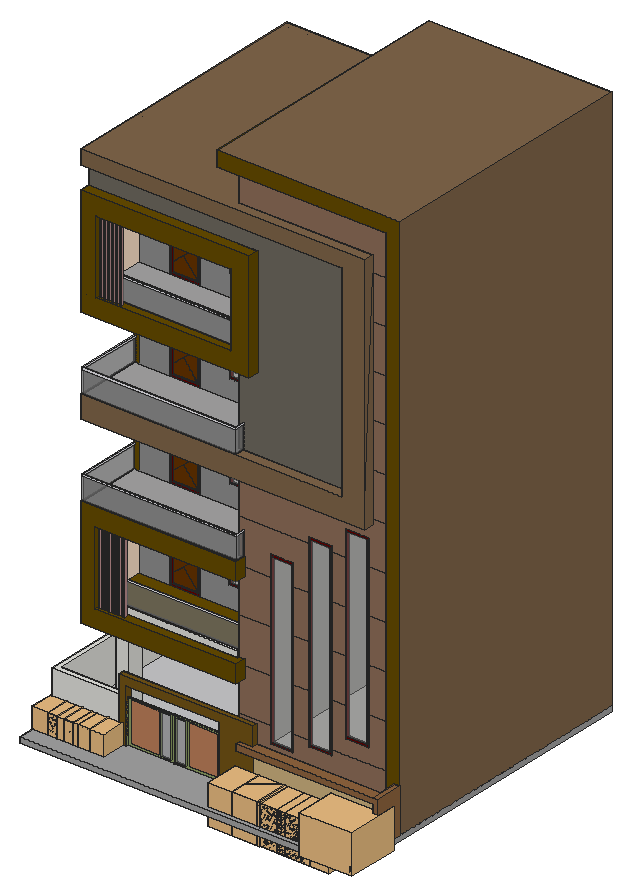
# SketchUp Ruby script. Lengths in inches.
U = 1.inch
M = Sketchup.active_model
def pt(a) = Geom::Point3d.new(a.map { |v| v * U })
def face(e, loops, mat)
  f = e.add_face(loops[0].map { |a| pt(a) })
  loops[1..].each { |l| e.add_face(l.map { |a| pt(a) }).erase! }
  f.material = f.back_material = mat if mat
  f
end
# faces: each face lists its corners as indices into pts; further lists are holes
def faces(e, pts, list, mat = nil) = list.each { |f| face(e, (f[0].is_a?(Array) ? f : [f]).map { |l| l.map { |i| pts[i] } }, mat) }
# xy, xz, yz: faces in a plane at the given z, y or x. An outline is a flat list of corners, or four numbers for a rectangle; further outlines are holes
def ring(l) = l.size == 4 ? [[l[0], l[1]], [l[2], l[1]], [l[2], l[3]], [l[0], l[3]]] : l.each_slice(2).to_a
def flat(e, list, mat, &to3) = list.each { |f| face(e, (f[0].is_a?(Array) ? f : [f]).map { |l| ring(l).map { |u, v| to3.(u, v) } }, mat) }
def xy(e, z, list, mat = nil) = flat(e, list, mat) { |x, y| [x, y, z] }
def xz(e, y, list, mat = nil) = flat(e, list, mat) { |x, z| [x, y, z] }
def yz(e, x, list, mat = nil) = flat(e, list, mat) { |y, z| [x, y, z] }
def lines(e, pts, list) = list.each { |a, b| e.add_line(pt(pts[a]), pt(pts[b])) }
# prism: a flat outline (further loops are holes) pulled along v
def prism(e, loops, v, mat = nil)
  f = face(e, loops, mat); d = Geom::Vector3d.new(v.map { |x| x * U })
  f.pushpull(f.normal.samedirection?(d) ? d.length : -d.length)
end
def box(e, o, s, mat = nil) = prism(e, [[o, [o[0] + s[0], o[1], o[2]], [o[0] + s[0], o[1] + s[1], o[2]], [o[0], o[1] + s[1], o[2]]]], [0, 0, s[2]], mat)
def at(x, y, z, deg = 0) = Geom::Transformation.translation(pt([x, y, z])) * Geom::Transformation.rotation(ORIGIN, Z_AXIS, deg.degrees)
def axes(o, x, y, z) = Geom::Transformation.new([*x, 0, *y, 0, *z, 0, *pt(o).to_a, 1])
def part(name) = M.definitions.add(name)
# library, detail: a bought-in or finely detailed component or shape, given as its bounding box
def library(name, o, s) = part(name).tap { |d| box(d.entities, o, s) }
def detail(e, o, s) = box(e.add_group.entities, o, s)
def put(e, d, t, mat = nil) = e.add_instance(d, t).tap { |i| i.material = mat if mat }
def group(e, t, mat = nil) = e.add_group.tap { |g| g.transformation = t; g.material = mat if mat }.entities
root = M.entities
M.materials.add("[0040_Peru]").color = [143, 110, 89]
M.materials.add("[0040_Peru]1").color = [143, 101, 63]
M.materials.add("[0040_Peru]2").color = [205, 133, 63]
M.materials.add("[0058_Olive]").color = [128, 102, 74]
M.materials.add("[0058_Olive]1").color = [143, 161, 101]
M.materials.add("[0058_Olive]2").color = [114, 83, 22]
M.materials.add("[0119_RosyBrown]").color = [188, 143, 143]
M.materials.add("[Blacktop Old 02]").color = [143, 145, 145]
M.materials.add("[Cladding Weathered]1").color = [111, 105, 96]
M.materials.add("[Color A08]").color = [102, 0, 0]
M.materials.add("[Color B08]").color = [102, 25, 0]
M.materials.add("[Color C01]").color = [255, 229, 204]
M.materials.add("[Color C08]").color = [102, 51, 0]
M.materials.add("[Color D08]").color = [102, 76, 0]
M.materials.add("[Color M04]").color = [142, 142, 142]
M.materials.add("[Grass Dark Green]").color = [106, 157, 55]
M.materials.add("[Metal Silver]").color = [234, 233, 238]
M.materials.add("[Pavers Flagstone Gray]").color = [162, 162, 162]
M.materials.add("[Polished Concrete New]").color = [200, 200, 203]
M.materials.add("[Stone Sandstone Ashlar Light]").color = [206, 178, 128]
M.materials.add("[Stone Vein Gray]").color = [166, 165, 165]
M.materials.add("[Translucent Glass Gray]").color = [128, 128, 128]
M.materials["[Translucent Glass Gray]"].alpha = 0.5
M.materials.add("[Wood Veneer 02]").color = [190, 128, 91]
c1 = library("Flowering shrub",[-7.36,-7.49,-12.9],[86.01,85.74,63.18])
c2 = library("plant\#1",[-28.7,-9.94,-2.13],[41.67,42.29,34.27])
c3 = part("Group\#2")
xy(c3.entities,0,[[0,0,52.4375,3.1875]],"[Color A08]")
xy(c3.entities,2.41,[[2.41,0,24.62,3.1875],[26.04,0,50.02,3.1875]],"[Color A08]")
xy(c3.entities,67.21,[[2.41,0,24.62,3.1875],[26.04,0,50.02,3.1875]],"[Color A08]")
xy(c3.entities,69.625,[[0,0,52.4375,3.1875]],"[Color A08]")
xz(c3.entities,0,[[[0,0,52.4375,69.625],[26.04,2.41,50.02,67.21],[2.41,2.41,24.62,67.21]]],"[Color A08]")
xz(c3.entities,0,[[2.41,2.41,24.62,67.21],[26.04,2.41,50.02,67.21]],"[Translucent Glass Gray]")
xz(c3.entities,3.1875,[[[0,0,52.4375,69.625],[26.04,2.41,50.02,67.21],[2.41,2.41,24.62,67.21]]],"[Color A08]")
yz(c3.entities,0,[[0,0,3.1875,69.625]],"[Color A08]")
yz(c3.entities,2.41,[[0,2.41,3.1875,67.21]],"[Color A08]")
yz(c3.entities,24.62,[[0,2.41,3.1875,67.21]],"[Color A08]")
yz(c3.entities,26.04,[[0,2.41,3.1875,67.21]],"[Color A08]")
yz(c3.entities,50.02,[[0,2.41,3.1875,67.21]],"[Color A08]")
yz(c3.entities,52.4375,[[0,0,3.1875,69.625]],"[Color A08]")
c4 = part("Group\#1")
xy(c4.entities,0,[[0,0,27.5625,2.875]],"[Color A08]")
xy(c4.entities,2.09,[[2.09,0,25.47,2.875]],"[Color A08]")
xy(c4.entities,198.72,[[2.09,0,25.47,2.875]],"[Color A08]")
xy(c4.entities,200.8125,[[0,0,27.5625,2.875]],"[Color A08]")
xz(c4.entities,0,[[[0,0,27.5625,200.8125],[2.09,2.09,25.47,198.72]]],"[Color A08]")
xz(c4.entities,0,[[2.09,2.09,25.47,198.72]],"[Translucent Glass Gray]")
xz(c4.entities,2.875,[[[0,0,27.5625,200.8125],[2.09,2.09,25.47,198.72]]],"[Color A08]")
yz(c4.entities,0,[[0,0,2.875,200.8125]],"[Color A08]")
yz(c4.entities,2.09,[[0,2.09,2.875,198.72]],"[Color A08]")
yz(c4.entities,25.47,[[0,2.09,2.875,198.72]],"[Color A08]")
yz(c4.entities,27.5625,[[0,0,2.875,200.8125]],"[Color A08]")
c5 = part("Group\#3")
xy(c5.entities,0,[[0,0,48,2.4375]],"[Color A08]")
xy(c5.entities,2.92,[[2.92,0,45.08,2.4375]],"[Color A08]")
xy(c5.entities,81.08,[[2.92,0,37.65,2.4375],[37.65,0,40.5,2.4375],[40.5,0,45.08,2.4375]],"[Color B08]")
xy(c5.entities,84,[[0,0,48,2.4375]],"[Color A08]")
xz(c5.entities,0,[[[0,0,48,84],[2.92,2.92,45.08,81.08]]],"[Color A08]")
xz(c5.entities,2.4375,[[43.2,2.92,45.08,2.92,20.8,32.14,38.67,46.92,45.08,39.74,45.08,42,23.56,65.96,40.5,81.08,37.65,81.08,2.92,50.08,2.92,47.53,22.51,65.02,37.92,47.76,2.92,18.84,2.92,17.37,20.04,31.52]])
xz(c5.entities,2.4375,[[[0,0,48,84],[2.92,2.92,45.08,81.08]]],"[Color A08]")
xz(c5.entities,2.4375,[[2.92,2.92,43.2,2.92,20.04,31.52,2.92,17.37],[45.08,2.92,45.08,39.74,38.67,46.92,20.8,32.14],[2.92,18.84,37.92,47.76,22.51,65.02,2.92,47.53],[45.08,42,45.08,81.08,40.5,81.08,23.56,65.96],[2.92,50.08,37.65,81.08,2.92,81.08]],"[Color C08]")
yz(c5.entities,0,[[0,0,2.4375,84]],"[Color A08]")
yz(c5.entities,2.92,[[0,2.92,2.4375,81.08]],"[Color A08]")
yz(c5.entities,45.08,[[0,2.92,2.4375,81.08]],"[Color B08]")
yz(c5.entities,48,[[0,0,2.4375,84]],"[Color A08]")
xy(root,0,[[0,0,537.625,532.0625]],"[Pavers Flagstone Gray]")
xy(root,9,[[[327.04,23.21,528.625,64.625],[330.38,27.13,524.7,60.7]],[528.625,56.9375,528.625,64.625,327.04,64.625,327.04,73.625,528.625,73.625,528.625,101.03,537.625,101.03,537.625,56.9375],[0,64.625,0,532.0625,9,532.0625,9,73.625,109.37,73.625,109.37,64.625],[109.37,64.625,121.05,73.625],[271.17,64.625,327.04,73.625],
  [515.375,101.03,515.375,128.4375,253.8125,128.4375,253.8125,523.0625,9,523.0625,9,532.0625,259.8125,532.0625,259.8125,134.4375,528.625,134.4375,528.625,532.0625,537.625,532.0625,537.625,101.03],[259.8125,134.4375,528.625,523.0625],[45.43,138.76,66.61,163.51],[45.43,291.51,66.61,316.26],[45.43,446.64,66.61,471.39],
  [259.8125,523.0625,528.625,532.0625]])
xy(root,9,[[330.38,27.13,524.7,60.7]],"[Grass Dark Green]")
xy(root,9,[[0,0,537.625,0,537.625,56.9375,528.625,56.9375,528.625,23.21,327.04,23.21,327.04,64.625,271.17,64.625,271.17,73.625,121.05,73.625,121.05,64.625,0,64.625]],"[Pavers Flagstone Gray]")
xy(root,9,[[[9,73.625,528.625,73.625,528.625,101.03,515.375,101.03,515.375,128.4375,253.8125,128.4375,253.8125,523.0625,9,523.0625],[45.43,138.76,66.61,163.51],[45.43,291.51,66.61,316.26],[45.43,446.64,66.61,471.39]]],"[Polished Concrete New]")
xy(root,24.25,[[[327.04,23.21,528.625,64.625],[330.38,27.13,524.7,60.7]]],"[0040_Peru]2")
xy(root,48.93,[[305.64,128.4375,342.2,134.4375]])
xy(root,66.76,[[368.38,128.4375,404.94,134.4375]])
xy(root,71.19,[[305.73,56.9375,327.04,64.625],[327.04,56.9375,528.625,64.625]],"[0040_Peru]1")
xy(root,81,[[0,64.625,109.37,64.625,109.37,73.625,9,73.625,9,532.0625,0,532.0625]])
xy(root,81,[[305.73,56.9375,528.625,56.9375,528.625,73.625,327.04,73.625,327.04,64.625,305.73,64.625],[528.625,56.9375,537.625,101.03]],"[0040_Peru]1")
xy(root,97.35,[[121.05,64.625,271.17,73.625]],"[0058_Olive]2")
xy(root,99.7,[[427.94,128.4375,464.51,134.4375]])
xy(root,110.8125,[[109.37,64.625,327.04,73.625]],"[0058_Olive]2")
xy(root,129,[[45.43,138.76,66.61,163.51],[45.43,291.51,66.61,316.26],[45.43,446.64,66.61,471.39]])
xy(root,129,[[9,111.5625,9,523.0625,253.8125,523.0625,253.8125,128.4375,262.75,128.4375,262.75,111.5625]],"[Blacktop Old 02]")
xy(root,141,[[18,134.4375,253.8125,523.0625]])
xy(root,158,[[32.1875,126.9375,253.76,132.4375],[18,134.4375,32.1875,140.99],[18,225.75,253.8125,523.0625]])
xy(root,158,[[34.74,117.78,38.43,121.47],[40.12,117.78,43.81,121.47],[45.49,117.78,49.18,121.47],[50.87,117.78,54.56,121.47],[56.24,117.78,59.93,121.47],
  [61.62,117.78,65.31,121.47],[66.99,117.78,70.68,121.47],[72.37,117.78,76.06,121.47]],"[0119_RosyBrown]")
xy(root,158,[[[32.1875,111.5625,262.75,111.5625,262.75,128.4375,253.8125,128.4375,253.8125,219.75,116.53,219.75,116.53,225.75,68.53,225.75,68.53,219.75,18,219.75,18,140.99,32.1875,140.99,32.1875,132.4375,253.76,132.4375,253.76,126.9375,32.1875,126.9375],[34.74,117.78,38.43,121.47],[40.12,117.78,43.81,121.47],[45.49,117.78,49.18,121.47],[50.87,117.78,54.56,121.47],[56.24,117.78,59.93,121.47],[61.62,117.78,65.31,121.47],[66.99,117.78,70.68,121.47],[72.37,117.78,76.06,121.47]]],"[Color D08]")
xy(root,168.0625,[[32.1875,126.9375,253.76,128.75],[32.1875,128.75,253.76,129.5],[32.1875,129.5,253.76,132.4375]])
xy(root,191.6,[[164.14,219.75,207.76,225.75]])
xy(root,204.0625,[[32.1875,128.75,253.76,129.5]],"[Metal Silver]")
xy(root,207.0625,[[32.1875,128.75,253.76,129.5]],"[Metal Silver]")
xy(root,242,[[68.53,219.75,116.53,225.75]])
xy(root,242.98,[[164.14,219.75,207.76,225.75]])
xy(root,278,[[[32.1875,111.5625,32.1875,140.99,18,140.99,18,219.75,253.8125,219.75,253.8125,128.4375,262.75,128.4375,262.75,111.5625],[34.74,117.78,38.43,121.47],[40.12,117.78,43.81,121.47],[45.49,117.78,49.18,121.47],[50.87,117.78,54.56,121.47],[56.24,117.78,59.93,121.47],[61.62,117.78,65.31,121.47],[66.99,117.78,70.68,121.47],[72.37,117.78,76.06,121.47]]],"[Color C01]")
xy(root,301.75,[[18,225.75,253.8125,523.0625]])
xy(root,307,[[9,111.5625,262.75,111.5625,262.75,128.4375,262,128.4375,262,114.0625,9.5625,114.0625,9.5625,219.75,9,219.75],[9.5625,114.0625,9.5625,219.75,11.5625,219.75,11.5625,115.25,260,115.25,260,128.4375,262,128.4375,262,114.0625],[68.53,219.75,116.53,225.75],[18,225.75,253.8125,523.0625]])
xy(root,307,[[11.5625,115.25,260,115.25,260,128.4375,253.8125,128.4375,253.8125,219.75,11.5625,219.75]],"[Stone Vein Gray]")
xy(root,325.79,[[305.64,128.4375,342.2,134.4375]])
xy(root,339.73,[[165.33,219.75,208.95,225.75]])
xy(root,343,[[9.5625,114.0625,9.5625,219.75,11.5625,219.75,11.5625,115.25,260,115.25,260,128.4375,262,128.4375,262,114.0625]],"[Metal Silver]")
xy(root,346,[[9.5625,114.0625,262,114.0625,262,128.4375,260,128.4375,260,115.25,11.5625,115.25,11.5625,219.75,9.5625,219.75]],"[Metal Silver]")
xy(root,373.01,[[368.38,128.4375,404.94,134.4375]])
xy(root,391,[[68.53,219.75,116.53,225.75]])
xy(root,391.1,[[165.33,219.75,208.95,225.75]])
xy(root,405.95,[[427.94,128.4375,464.51,134.4375]])
xy(root,427,[[9,111.5625,9,219.75,253.8125,219.75,253.8125,128.4375,471.49,128.4375,471.49,111.5625]],"[0058_Olive]")
xy(root,454.25,[[18,225.75,253.8125,523.0625]])
xy(root,457,[[259.8125,134.4375,528.625,523.0625]])
xy(root,463,[[9.875,112.5,9.875,219.75,11.875,219.75,11.875,114.5,259.59,114.5,259.59,128.4375,261.59,128.4375,261.59,112.5],[259.8125,134.4375,528.625,523.0625],[68.53,219.75,116.53,225.75],[18,225.75,253.8125,523.0625]])
xy(root,463,[[9,111.5625,434.21,111.5625,434.21,128.4375,261.59,128.4375,261.59,112.5,9.875,112.5,9.875,219.75,9,219.75]],"[0058_Olive]")
xy(root,463,[[11.875,114.5,259.59,114.5,259.59,128.4375,253.8125,128.4375,253.8125,219.75,11.875,219.75]],"[Stone Vein Gray]")
xy(root,493.41,[[165.33,219.75,208.95,225.75]])
xy(root,499,[[9.875,112.5,9.875,219.75,11.875,219.75,11.875,114.5,259.59,114.5,259.59,128.4375,261.59,128.4375,261.59,112.5]],"[Metal Silver]")
xy(root,502,[[9.875,112.5,261.59,112.5,261.59,128.4375,259.59,128.4375,259.59,114.5,11.875,114.5,11.875,219.75,9.875,219.75]],"[Metal Silver]")
xy(root,544.79,[[165.33,219.75,208.95,225.75]])
xy(root,548.125,[[68.53,219.75,116.53,225.75]])
xy(root,583,[[9,111.5625,9,219.75,253.8125,219.75,253.8125,128.4375,283.75,128.4375,283.75,111.5625]],"[Color D08]")
xy(root,606,[[18,225.75,253.8125,523.0625]])
xy(root,607,[[259.8125,134.4375,528.625,523.0625]])
xy(root,612,[[34.5625,124.3125,253.8125,126.3125],[259.8125,134.4375,528.625,523.0625],[68.53,219.75,116.53,225.75],[18,225.75,253.8125,523.0625]])
xy(root,612,[[36.42,116.43,39.73,120.18],[42.85,116.43,46.17,120.18],[49.29,116.43,52.6,120.18],[55.73,116.43,59.04,120.18],[62.17,116.43,65.48,120.18],
  [68.6,116.43,71.92,120.18]],"[0119_RosyBrown]")
xy(root,612,[[[34.5625,111.5625,253.8125,124.3125],[36.42,116.43,39.73,120.18],[42.85,116.43,46.17,120.18],[49.29,116.43,52.6,120.18],[55.73,116.43,59.04,120.18],[62.17,116.43,65.48,120.18],[68.6,116.43,71.92,120.18]]],"[Color D08]")
xy(root,612,[[34.5625,126.3125,253.8125,126.3125,253.8125,219.75,18,219.75,18,133.33,34.5625,133.33]],"[Stone Vein Gray]")
xy(root,647.35,[[165.33,219.75,208.95,225.75]])
xy(root,648,[[34.5625,124.3125,253.8125,126.3125]],"[Metal Silver]")
xy(root,651,[[34.5625,124.3125,253.8125,126.3125]],"[Metal Silver]")
xy(root,696.6875,[[68.53,219.75,116.53,225.75]])
xy(root,698.73,[[165.33,219.75,208.95,225.75]])
xy(root,732,[[[34.5625,111.5625,34.5625,133.33,18,133.33,18,219.75,253.8125,219.75,253.8125,111.5625],[36.42,116.43,39.73,120.18],[42.85,116.43,46.17,120.18],[49.29,116.43,52.6,120.18],[55.73,116.43,59.04,120.18],[62.17,116.43,65.48,120.18],[68.6,116.43,71.92,120.18]]],"[Color C01]")
xy(root,761,[[9,111.5625,283.75,128.4375]],"[Color D08]")
xy(root,797,[[9,111.5625,434.21,128.4375]])
xy(root,809,[[259.8125,134.4375,528.625,523.0625],[18,225.75,253.8125,523.0625]])
xy(root,821,[[259.8125,134.4375,528.625,523.0625],[259.8125,134.4375,528.625,523.0625]])
xy(root,821,[[9,111.5625,471.49,111.5625,471.49,128.4375,253.8125,128.4375,253.8125,532.0625,9,532.0625]],"[0058_Olive]")
xy(root,881,[[240.125,101.03,253.8125,532.0625],[253.8125,101.03,515.375,128.4375]],"[Color D08]")
xy(root,905,[[240.125,101.03,537.625,532.0625]],"[0058_Olive]")
xz(root,0,[[0,0,537.625,9]],"[Pavers Flagstone Gray]")
xz(root,23.21,[[327.04,9,528.625,24.25]],"[0040_Peru]2")
xz(root,27.13,[[330.38,9,524.7,24.25]],"[0040_Peru]2")
xz(root,56.9375,[[528.625,9,537.625,9,537.625,81,305.73,81,305.73,71.19,528.625,71.19]],"[0040_Peru]1")
xz(root,60.7,[[330.38,9,524.7,24.25]],"[0040_Peru]2")
xz(root,64.625,[[0,9,109.37,81],[327.04,9,528.625,24.25]])
xz(root,64.625,[[109.37,9,121.05,9,121.05,97.35,271.17,97.35,271.17,9,327.04,9,327.04,71.19,305.73,71.19,305.73,81,327.04,81,327.04,110.8125,109.37,110.8125]],"[0058_Olive]2")
xz(root,64.625,[[327.04,24.25,528.625,71.19]],"[Stone Sandstone Ashlar Light]")
xz(root,73.625,[[9,9,109.37,81]])
xz(root,73.625,[[327.04,9,528.625,81]],"[0040_Peru]1")
xz(root,73.625,[[109.37,9,109.37,110.8125,327.04,110.8125,327.04,9,271.17,9,271.17,97.35,121.05,97.35,121.05,9]],"[0058_Olive]2")
xz(root,101.03,[[528.625,9,537.625,81]])
xz(root,101.03,[[515.375,9,528.625,9,528.625,81,537.625,81,537.625,905,240.125,905,240.125,881,515.375,881]],"[Color D08]")
xz(root,111.5625,[[9,427,471.49,427,471.49,821,9,821,9,797,434.21,797,434.21,463,9,463]],"[0058_Olive]")
xz(root,111.5625,[[9,129,262.75,129,262.75,158,32.1875,158,32.1875,278,262.75,278,262.75,307,9,307],[[9,583,283.75,761],[34.5625,612,253.8125,732]]],"[Color D08]")
xz(root,112.5,[[9.875,499,261.59,502]],"[Metal Silver]")
xz(root,112.5,[[9.875,463,261.59,499]],"[Translucent Glass Gray]")
xz(root,114.0625,[[9.5625,343,262,346]],"[Metal Silver]")
xz(root,114.0625,[[9.5625,307,262,343]],"[Translucent Glass Gray]")
xz(root,114.5,[[11.875,499,259.59,502]],"[Metal Silver]")
xz(root,114.5,[[11.875,463,259.59,499]],"[Translucent Glass Gray]")
xz(root,115.25,[[11.5625,343,260,346]],"[Metal Silver]")
xz(root,115.25,[[11.5625,307,260,343]],"[Translucent Glass Gray]")
xz(root,116.43,[[36.42,612,39.73,732],[42.85,612,46.17,732],[49.29,612,52.6,732],[55.73,612,59.04,732],[62.17,612,65.48,732],
  [68.6,612,71.92,732]],"[0119_RosyBrown]")
xz(root,117.78,[[34.74,158,38.43,278],[40.12,158,43.81,278],[45.49,158,49.18,278],[50.87,158,54.56,278],[56.24,158,59.93,278],
  [61.62,158,65.31,278],[66.99,158,70.68,278],[72.37,158,76.06,278]],"[0119_RosyBrown]")
xz(root,120.18,[[36.42,612,39.73,732],[42.85,612,46.17,732],[49.29,612,52.6,732],[55.73,612,59.04,732],[62.17,612,65.48,732],
  [68.6,612,71.92,732]],"[0119_RosyBrown]")
xz(root,121.47,[[34.74,158,38.43,278],[40.12,158,43.81,278],[45.49,158,49.18,278],[50.87,158,54.56,278],[56.24,158,59.93,278],
  [61.62,158,65.31,278],[66.99,158,70.68,278],[72.37,158,76.06,278]],"[0119_RosyBrown]")
xz(root,124.3125,[[34.5625,648,253.8125,651]],"[Metal Silver]")
xz(root,124.3125,[[34.5625,612,253.8125,648]],"[Translucent Glass Gray]")
xz(root,126.3125,[[34.5625,648,253.8125,651]],"[Metal Silver]")
xz(root,126.3125,[[34.5625,612,253.8125,648]],"[Translucent Glass Gray]")
xz(root,126.9375,[[32.1875,158,253.76,168.0625]])
xz(root,128.4375,[[253.8125,278,262.75,307],[260,307,262,343],[253.8125,427,253.8125,463,434.21,463,434.21,797,253.8125,797,253.8125,821,471.49,821,471.49,427],[259.59,463,261.59,499],[253.8125,583,283.75,612],
  [253.8125,732,283.75,761]])
xz(root,128.4375,[[253.8125,9,515.375,9,515.375,76.28,404.94,76.28,404.94,66.76,368.38,66.76,368.38,76.28,342.2,76.28,342.2,48.93,305.64,48.93,305.64,76.28,253.8125,76.28],[253.8125,76.28,305.64,76.28,305.64,148.21,262.75,148.21,262.75,129,253.8125,129],[342.2,76.28,368.38,148.21],[404.94,76.28,515.375,76.28,515.375,148.21,464.51,148.21,464.51,99.7,427.94,99.7,427.94,148.21,404.94,148.21],[262.75,148.21,305.64,148.21,305.64,220.15,253.8125,220.15,253.8125,158,262.75,158],
  [342.2,148.21,368.38,220.15],[404.94,148.21,427.94,220.15],[464.51,148.21,515.375,220.15],[253.8125,220.15,305.64,220.15,305.64,292.09,262.75,292.09,262.75,278,253.8125,278],[342.2,220.15,368.38,292.09],
  [404.94,220.15,427.94,292.09],[464.51,220.15,515.375,292.09],[262.75,292.09,305.64,292.09,305.64,325.79,342.2,325.79,342.2,292.09,368.38,292.09,368.38,364.03,253.8125,364.03,253.8125,307,260,307,260,346,262,346,262,307,262.75,307],[404.94,292.09,427.94,364.03],[464.51,292.09,515.375,364.03],
  [253.8125,364.03,368.38,364.03,368.38,373.01,404.94,373.01,404.94,364.03,427.94,364.03,427.94,405.95,464.51,405.95,464.51,364.03,515.375,364.03,515.375,435.96,471.49,435.96,471.49,427,253.8125,427],[471.49,435.96,515.375,507.9],[471.49,507.9,515.375,579.84],[471.49,579.84,515.375,651.78],[471.49,651.78,515.375,723.71],
  [471.49,723.71,515.375,795.65],[471.49,795.65,515.375,795.65,515.375,881,253.8125,881,253.8125,821,471.49,821]],"[0040_Peru]")
xz(root,128.4375,[[253.8125,463,259.59,463,259.59,502,261.59,502,261.59,463,434.21,463,434.21,797,9,797,9,761,283.75,761,283.75,583,253.8125,583]],"[Cladding Weathered]1")
xz(root,128.4375,[[260,343,262,346],[259.59,499,261.59,502]],"[Metal Silver]")
xz(root,128.75,[[32.1875,204.0625,253.76,207.0625]],"[Metal Silver]")
xz(root,128.75,[[32.1875,168.0625,253.76,204.0625]],"[Translucent Glass Gray]")
xz(root,129.5,[[32.1875,204.0625,253.76,207.0625]],"[Metal Silver]")
xz(root,129.5,[[32.1875,168.0625,253.76,204.0625]],"[Translucent Glass Gray]")
xz(root,132.4375,[[32.1875,158,253.76,168.0625]])
xz(root,133.33,[[18,612,34.5625,732]])
xz(root,134.4375,[[[259.8125,9,528.625,427],[368.38,66.76,404.94,373.01],[427.94,99.7,464.51,405.95],[305.64,48.93,342.2,325.79]],[259.8125,427,528.625,457],[259.8125,457,528.625,463],[259.8125,463,528.625,583],[259.8125,583,528.625,607],
  [259.8125,607,528.625,612],[259.8125,612,528.625,809],[259.8125,809,528.625,821]])
xz(root,138.76,[[45.43,9,66.61,129]])
xz(root,140.99,[[18,158,32.1875,278]])
xz(root,163.51,[[45.43,9,66.61,129]])
xz(root,219.75,[[18,278,253.8125,307],[9.5625,307,11.5625,343],[9.875,463,11.875,499]])
xz(root,219.75,[[9,307,9.5625,307,9.5625,346,11.5625,346,11.5625,307,18,307,18,427,9,427],[9,463,9.875,463,9.875,502,11.875,502,11.875,463,18,463,18,583,9,583]],"[Color D08]")
xz(root,219.75,[[[18,158,68.53,158,68.53,242,116.53,242,116.53,158,253.8125,158,253.8125,278,18,278],[164.14,191.6,207.76,242.98]],[[18,307,68.53,307,68.53,391,116.53,391,116.53,307,253.8125,307,253.8125,427,18,427],[165.33,339.73,208.95,391.1]],[[18,463,68.53,463,68.53,548.125,116.53,548.125,116.53,463,253.8125,463,253.8125,583,18,583],[165.33,493.41,208.95,544.79]],[[18,612,68.53,612,68.53,696.6875,116.53,696.6875,116.53,612,253.8125,612,253.8125,732,18,732],[165.33,647.35,208.95,698.73]]],"[Color M04]")
xz(root,219.75,[[9.5625,343,11.5625,346],[9.875,499,11.875,502]],"[Metal Silver]")
xz(root,225.75,[[[18,158,18,278,253.8125,278,253.8125,158,116.53,158,116.53,242,68.53,242,68.53,158],[164.14,191.6,207.76,242.98]],[18,278,253.8125,301.75],[18,301.75,68.53,307],[68.53,301.75,116.53,307],[116.53,301.75,253.8125,307],
  [[18,307,18,427,253.8125,427,253.8125,307,116.53,307,116.53,391,68.53,391,68.53,307],[165.33,339.73,208.95,391.1]],[18,427,253.8125,454.25],[18,454.25,68.53,463],[68.53,454.25,116.53,463],[116.53,454.25,253.8125,463],
  [[18,463,18,583,253.8125,583,253.8125,463,116.53,463,116.53,548.125,68.53,548.125,68.53,463],[165.33,493.41,208.95,544.79]],[18,583,253.8125,606],[18,606,68.53,612],[68.53,606,116.53,612],[116.53,606,253.8125,612],
  [[18,612,18,732,253.8125,732,253.8125,612,116.53,612,116.53,696.6875,68.53,696.6875,68.53,612],[165.33,647.35,208.95,698.73]],[18,732,253.8125,761],[18,761,253.8125,797],[18,797,253.8125,809]])
xz(root,291.51,[[45.43,9,66.61,129]])
xz(root,316.26,[[45.43,9,66.61,129]])
xz(root,446.64,[[45.43,9,66.61,129]])
xz(root,471.39,[[45.43,9,66.61,129]])
xz(root,523.0625,[[259.8125,9,528.625,427],[18,141,253.8125,158],[18,158,253.8125,278],[18,278,253.8125,301.75],[18,301.75,135.91,307],
  [135.91,301.75,148.84,307],[148.84,301.75,253.8125,307],[18,307,253.8125,427],[18,427,253.8125,454.25],[259.8125,427,528.625,457],
  [18,454.25,35.25,463],[35.25,454.25,72,463],[72,454.25,253.8125,463],[259.8125,457,295.61,463],[295.61,457,311.42,463],
  [311.42,457,528.625,463],[18,463,253.8125,583],[259.8125,463,528.625,583],[18,583,253.8125,606],[259.8125,583,528.625,607],
  [18,606,60.84,612],[60.84,606,68.27,612],[68.27,606,253.8125,612],[259.8125,607,279.55,612],[279.55,607,296.11,612],
  [296.11,607,528.625,612],[18,612,253.8125,809],[259.8125,612,528.625,809],[259.8125,809,266.0625,821],[266.0625,809,528.625,821]])
xz(root,523.0625,[[9,9,253.8125,129]],"[Blacktop Old 02]")
xz(root,532.0625,[[0,9,9,81]])
xz(root,532.0625,[[9,9,9,821,253.8125,821,253.8125,881,240.125,881,240.125,905,537.625,905,537.625,9]],"[0058_Olive]")
xz(root,532.0625,[[0,0,537.625,9]],"[Pavers Flagstone Gray]")
yz(root,0,[[64.625,9,532.0625,81]])
yz(root,0,[[0,0,532.0625,9]],"[Pavers Flagstone Gray]")
yz(root,9,[[73.625,9,523.0625,81],[523.0625,9,532.0625,81],[523.0625,81,532.0625,129]])
yz(root,9,[[111.5625,129,111.5625,307,219.75,307,219.75,427,111.5625,427,111.5625,463,219.75,463,219.75,583,111.5625,583,111.5625,761,128.4375,761,128.4375,797,111.5625,797,111.5625,821,532.0625,821,532.0625,129]],"[0058_Olive]")
yz(root,9.5625,[[114.0625,343,219.75,346]],"[Metal Silver]")
yz(root,9.5625,[[114.0625,307,219.75,343]],"[Translucent Glass Gray]")
yz(root,9.875,[[112.5,499,219.75,502]],"[Metal Silver]")
yz(root,9.875,[[112.5,463,219.75,499]],"[Translucent Glass Gray]")
yz(root,11.5625,[[115.25,343,219.75,346]],"[Metal Silver]")
yz(root,11.5625,[[115.25,307,219.75,343]],"[Translucent Glass Gray]")
yz(root,11.875,[[114.5,499,219.75,502]],"[Metal Silver]")
yz(root,11.875,[[114.5,463,219.75,499]],"[Translucent Glass Gray]")
yz(root,18,[[225.75,158,523.0625,278],[225.75,278,523.0625,301.75],[225.75,301.75,523.0625,307],[225.75,307,523.0625,427],[225.75,427,523.0625,454.25],
  [225.75,454.25,523.0625,463],[225.75,463,523.0625,583],[225.75,583,523.0625,606],[225.75,606,523.0625,612],[225.75,612,523.0625,809]])
yz(root,18,[[140.99,158,219.75,278],[133.33,612,219.75,732]],"[Color C01]")
yz(root,32.1875,[[126.9375,158,132.4375,168.0625],[128.75,168.0625,129.5,204.0625]])
yz(root,32.1875,[[111.5625,158,126.9375,158,126.9375,168.0625,128.75,168.0625,128.75,207.0625,129.5,207.0625,129.5,168.0625,132.4375,168.0625,132.4375,158,140.99,158,140.99,278,111.5625,278]],"[Color D08]")
yz(root,32.1875,[[128.75,204.0625,129.5,207.0625]],"[Metal Silver]")
yz(root,34.5625,[[124.3125,612,126.3125,648]])
yz(root,34.5625,[[111.5625,612,124.3125,612,124.3125,651,126.3125,651,126.3125,612,133.33,612,133.33,732,111.5625,732]],"[Color D08]")
yz(root,34.5625,[[124.3125,648,126.3125,651]],"[Metal Silver]")
yz(root,34.74,[[117.78,158,121.47,278]],"[0119_RosyBrown]")
yz(root,36.42,[[116.43,612,120.18,732]],"[0119_RosyBrown]")
yz(root,38.43,[[117.78,158,121.47,278]],"[0119_RosyBrown]")
yz(root,39.73,[[116.43,612,120.18,732]],"[0119_RosyBrown]")
yz(root,40.12,[[117.78,158,121.47,278]],"[0119_RosyBrown]")
yz(root,42.85,[[116.43,612,120.18,732]],"[0119_RosyBrown]")
yz(root,43.81,[[117.78,158,121.47,278]],"[0119_RosyBrown]")
yz(root,45.43,[[138.76,9,163.51,129],[291.51,9,316.26,129],[446.64,9,471.39,129]])
yz(root,45.49,[[117.78,158,121.47,278]],"[0119_RosyBrown]")
yz(root,46.17,[[116.43,612,120.18,732]],"[0119_RosyBrown]")
yz(root,49.18,[[117.78,158,121.47,278]],"[0119_RosyBrown]")
yz(root,49.29,[[116.43,612,120.18,732]],"[0119_RosyBrown]")
yz(root,50.87,[[117.78,158,121.47,278]],"[0119_RosyBrown]")
yz(root,52.6,[[116.43,612,120.18,732]],"[0119_RosyBrown]")
yz(root,54.56,[[117.78,158,121.47,278]],"[0119_RosyBrown]")
yz(root,55.73,[[116.43,612,120.18,732]],"[0119_RosyBrown]")
yz(root,56.24,[[117.78,158,121.47,278]],"[0119_RosyBrown]")
yz(root,59.04,[[116.43,612,120.18,732]],"[0119_RosyBrown]")
yz(root,59.93,[[117.78,158,121.47,278]],"[0119_RosyBrown]")
yz(root,61.62,[[117.78,158,121.47,278]],"[0119_RosyBrown]")
yz(root,62.17,[[116.43,612,120.18,732]],"[0119_RosyBrown]")
yz(root,65.31,[[117.78,158,121.47,278]],"[0119_RosyBrown]")
yz(root,65.48,[[116.43,612,120.18,732]],"[0119_RosyBrown]")
yz(root,66.61,[[138.76,9,163.51,129],[291.51,9,316.26,129],[446.64,9,471.39,129]])
yz(root,66.99,[[117.78,158,121.47,278]],"[0119_RosyBrown]")
yz(root,68.53,[[219.75,158,225.75,242],[219.75,307,225.75,391],[219.75,463,225.75,548.125],[219.75,612,225.75,696.6875]])
yz(root,68.6,[[116.43,612,120.18,732]],"[0119_RosyBrown]")
yz(root,70.68,[[117.78,158,121.47,278]],"[0119_RosyBrown]")
yz(root,71.92,[[116.43,612,120.18,732]],"[0119_RosyBrown]")
yz(root,72.37,[[117.78,158,121.47,278]],"[0119_RosyBrown]")
yz(root,76.06,[[117.78,158,121.47,278]],"[0119_RosyBrown]")
yz(root,109.37,[[64.625,9,73.625,81]])
yz(root,109.37,[[64.625,81,73.625,110.8125]],"[0058_Olive]2")
yz(root,116.53,[[219.75,158,225.75,242],[219.75,307,225.75,391],[219.75,463,225.75,548.125],[219.75,612,225.75,696.6875]])
yz(root,121.05,[[64.625,9,73.625,97.35]],"[0058_Olive]2")
yz(root,164.14,[[219.75,191.6,225.75,242.98]])
yz(root,165.33,[[219.75,339.73,225.75,391.1],[219.75,493.41,225.75,544.79],[219.75,647.35,225.75,698.73]])
yz(root,207.76,[[219.75,191.6,225.75,242.98]])
yz(root,208.95,[[219.75,339.73,225.75,391.1],[219.75,493.41,225.75,544.79],[219.75,647.35,225.75,698.73]])
yz(root,240.125,[[101.03,881,532.0625,905]],"[Color D08]")
yz(root,253.76,[[126.9375,158,132.4375,168.0625],[128.75,168.0625,129.5,204.0625]])
yz(root,253.76,[[128.75,204.0625,129.5,207.0625]],"[Metal Silver]")
yz(root,253.8125,[[134.4375,141,134.4375,158,219.75,158,219.75,821,225.75,821,225.75,158,523.0625,158,523.0625,141],[225.75,158,523.0625,278],[128.4375,278,134.4375,307],[134.4375,278,219.75,307],[225.75,278,523.0625,301.75],
  [225.75,301.75,523.0625,307],[225.75,307,523.0625,427],[128.4375,427,134.4375,463],[134.4375,427,219.75,463],[225.75,427,523.0625,454.25],
  [225.75,454.25,523.0625,463],[225.75,463,523.0625,583],[128.4375,583,134.4375,612],[134.4375,583,219.75,612],[225.75,583,523.0625,606],
  [225.75,606,523.0625,612],[124.3125,612,126.3125,648],[225.75,612,523.0625,809],[128.4375,732,134.4375,761],[134.4375,732,219.75,761],
  [128.4375,797,134.4375,821],[134.4375,797,219.75,821],[225.75,809,523.0625,821]])
yz(root,253.8125,[[128.4375,9,523.0625,129],[128.4375,158,219.75,278],[128.4375,307,219.75,427],[128.4375,463,219.75,583],[111.5625,612,111.5625,732,219.75,732,219.75,612,126.3125,612,126.3125,651,124.3125,651,124.3125,612],
  [128.4375,821,532.0625,881]],"[0040_Peru]")
yz(root,253.8125,[[124.3125,648,126.3125,651]],"[Metal Silver]")
yz(root,259.59,[[114.5,499,128.4375,502]],"[Metal Silver]")
yz(root,259.59,[[114.5,463,128.4375,499]],"[Translucent Glass Gray]")
yz(root,259.8125,[[134.4375,9,523.0625,427],[134.4375,427,523.0625,457],[134.4375,457,523.0625,463],[134.4375,463,523.0625,583],[134.4375,583,523.0625,607],
  [134.4375,607,523.0625,612],[134.4375,612,523.0625,809],[134.4375,809,523.0625,821]])
yz(root,260,[[115.25,343,128.4375,346]],"[Metal Silver]")
yz(root,260,[[115.25,307,128.4375,343]],"[Translucent Glass Gray]")
yz(root,261.59,[[112.5,499,128.4375,502]],"[Metal Silver]")
yz(root,261.59,[[112.5,463,128.4375,499]],"[Translucent Glass Gray]")
yz(root,262,[[114.0625,343,128.4375,346]],"[Metal Silver]")
yz(root,262,[[114.0625,307,128.4375,343]],"[Translucent Glass Gray]")
yz(root,262.75,[[111.5625,129,128.4375,158],[111.5625,278,128.4375,307]],"[Color D08]")
yz(root,271.17,[[64.625,9,73.625,97.35]],"[0058_Olive]2")
yz(root,283.75,[[111.5625,583,128.4375,761]],"[Color D08]")
yz(root,305.64,[[128.4375,48.93,134.4375,325.79]])
yz(root,305.73,[[56.9375,71.19,64.625,81]],"[0040_Peru]1")
yz(root,327.04,[[23.21,9,64.625,24.25]],"[0040_Peru]2")
yz(root,327.04,[[64.625,81,73.625,110.8125]],"[0058_Olive]2")
yz(root,330.38,[[27.13,9,60.7,24.25]],"[0040_Peru]2")
yz(root,342.2,[[128.4375,48.93,134.4375,325.79]])
yz(root,368.38,[[128.4375,66.76,134.4375,373.01]])
yz(root,404.94,[[128.4375,66.76,134.4375,373.01]])
yz(root,427.94,[[128.4375,99.7,134.4375,405.95]])
yz(root,434.21,[[111.5625,463,128.4375,797]],"[0058_Olive]")
yz(root,464.51,[[128.4375,99.7,134.4375,405.95]])
yz(root,471.49,[[111.5625,427,128.4375,427,128.4375,795.65,111.5625,463],[111.5625,463,128.4375,795.65,128.4375,821,111.5625,821]],"[0058_Olive]")
yz(root,515.375,[[101.03,9,128.4375,881]],"[Color D08]")
yz(root,524.7,[[27.13,9,56.9375,24.25],[56.9375,9,60.7,24.25]],"[0040_Peru]2")
yz(root,528.625,[[56.9375,9,64.625,24.25],[134.4375,9,523.0625,427],[134.4375,427,523.0625,457],[134.4375,457,523.0625,463],[134.4375,463,523.0625,583],
  [134.4375,583,523.0625,607],[134.4375,607,523.0625,612],[134.4375,612,523.0625,809],[134.4375,809,523.0625,821]])
yz(root,528.625,[[73.625,9,101.03,81],[56.9375,24.25,64.625,71.19]],"[0040_Peru]1")
yz(root,528.625,[[23.21,9,56.9375,24.25]],"[0040_Peru]2")
yz(root,537.625,[[56.9375,9,101.03,81]],"[0040_Peru]1")
yz(root,537.625,[[101.03,9,532.0625,905]],"[0058_Olive]")
yz(root,537.625,[[0,0,532.0625,9]],"[Pavers Flagstone Gray]")
p = [[18,134.4375,141],[18,134.4375,158],[528.625,523.0625,129],[528.625,532.0625,129],[9,219.75,797],[253.8125,219.75,797],
  [528.625,523.0625,463],[528.625,532.0625,463],[259.8125,523.0625,463],[259.8125,532.0625,463],[259.8125,523.0625,583],[259.8125,532.0625,583],
  [18,219.75,158],[9,219.75,158],[18,128.4375,158],[18,219.75,612],[9,219.75,612],[18,219.75,732],
  [9,219.75,732],[18,133.33,612],[18,111.5625,612],[49.6875,523.0625,821],[49.6875,523.0625,809],[18,225.75,809],
  [18,225.75,821],[18,523.0625,809],[18,523.0625,821],[259.8125,523.0625,821],[253.8125,523.0625,821]]
lines(root,p,[[0,1],[2,3],[4,5],[6,7],[8,9],[10,11],[12,13],[1,14],[15,16],[17,18],[19,20],[21,22],
  [23,24],[25,26],[27,28]])
put(root,c1,at(306.02,15.58,-6.875))
put(root,c1,at(345.21,15.58,-6.875))
put(root,c1,at(386.65,15.58,-6.875))
put(root,c1,at(418.34,15.58,-6.875))
put(root,c1,at(462.08,6.71,8.31))
put(root,c2,at(26.6,35.9,9))
put(root,c2,at(52.47,35.9,9))
put(root,c2,at(79.16,35.9,9))
put(root,c2,at(101.97,35.9,9))
put(root,c3,axes([164.14,220.71,191.6],[0.83194,0,0],[0,0.7,0],[0,0,0.73788]))
put(root,c4,axes([304.87,128.4375,48.93],[1.3545,0,0],[0,1,0],[0,0,1.37873]))
put(root,c4,axes([367.61,128.4375,66.76],[1.3545,0,0],[0,1,0],[0,0,1.52505]),"[Wood Veneer 02]")
put(root,c4,axes([427.17,128.4375,99.7],[1.3545,0,0],[0,1,0],[0,0,1.52505]))
put(root,c3,axes([165.33,220.71,339.73],[0.83194,0,0],[0,0.7,0],[0,0,0.73788]))
put(root,c3,axes([165.33,220.71,493.41],[0.83194,0,0],[0,0.7,0],[0,0,0.73788]))
put(root,c3,axes([165.33,220.71,647.35],[0.83194,0,0],[0,0.7,0],[0,0,0.73788]))
put(root,c5,at(68.53,219.75,158))
put(root,c5,at(68.53,219.75,307))
put(root,c5,axes([68.53,219.75,463],[1,0,0],[0,1,0],[0,0,1.01]))
put(root,c5,axes([68.53,219.75,612],[1,0,0],[0,1,0],[0,0,1.01]))
g1 = group(root,at(121.05,66.625,9))
xy(g1,0,[[0,0,74.14,1.85],[74.14,0,75.77,1.85],[75.77,0,150.11,1.85]],"[0058_Olive]1")
xy(g1,3.27,[[54.55,0,70.83,1.85],[79.29,0,95.67,1.85]],"[0058_Olive]1")
xy(g1,68.51,[[54.55,0,70.83,1.85],[79.29,0,95.67,1.85]],"[0058_Olive]1")
xy(g1,71.78,[[0,0,74.14,1.85],[74.14,0,75.77,1.85],[75.77,0,150.11,1.85]],"[0058_Olive]1")
xz(g1,0,[[54.55,3.27,70.83,68.51],[79.29,3.27,95.67,68.51]],"[Translucent Glass Gray]")
xz(g1,1.85,[[[0,0,74.14,71.78],[4.23,3.27,51.85,68.51],[54.55,3.27,70.83,68.51]],[74.14,0,75.77,71.78],[[75.77,0,150.11,71.78],[98.37,3.27,145.88,68.51],[79.29,3.27,95.67,68.51]]],"[0058_Olive]1")
xz(g1,1.85,[[4.23,3.27,51.85,68.51],[98.37,3.27,145.88,68.51]],"[Wood Veneer 02]")
yz(g1,0,[[0,0,1.85,71.78]],"[0058_Olive]1")
yz(g1,54.55,[[0,3.27,1.85,68.51]],"[0058_Olive]1")
yz(g1,70.83,[[0,3.27,1.85,68.51]],"[0058_Olive]1")
yz(g1,79.29,[[0,3.27,1.85,68.51]],"[0058_Olive]1")
yz(g1,95.67,[[0,3.27,1.85,68.51]],"[0058_Olive]1")
yz(g1,150.11,[[0,0,1.85,71.78]],"[0058_Olive]1")
